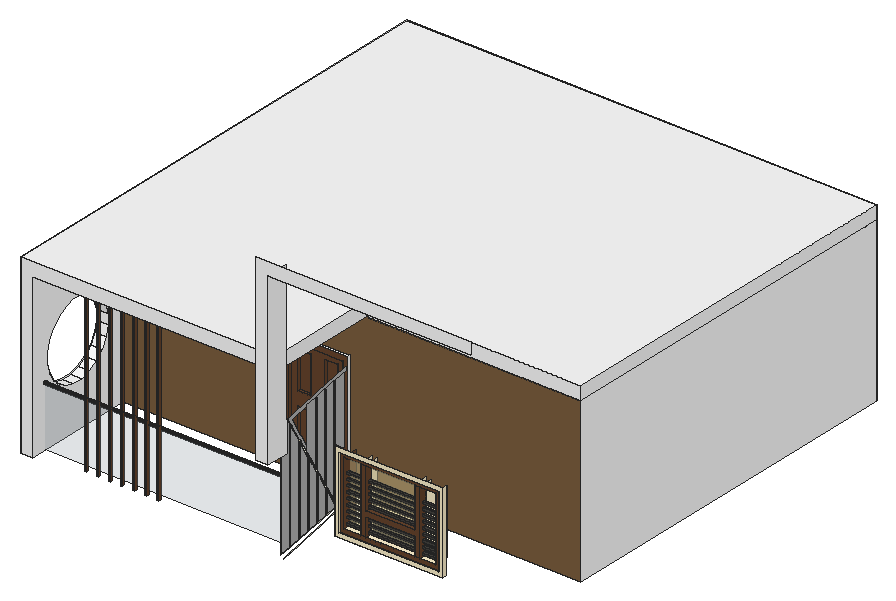
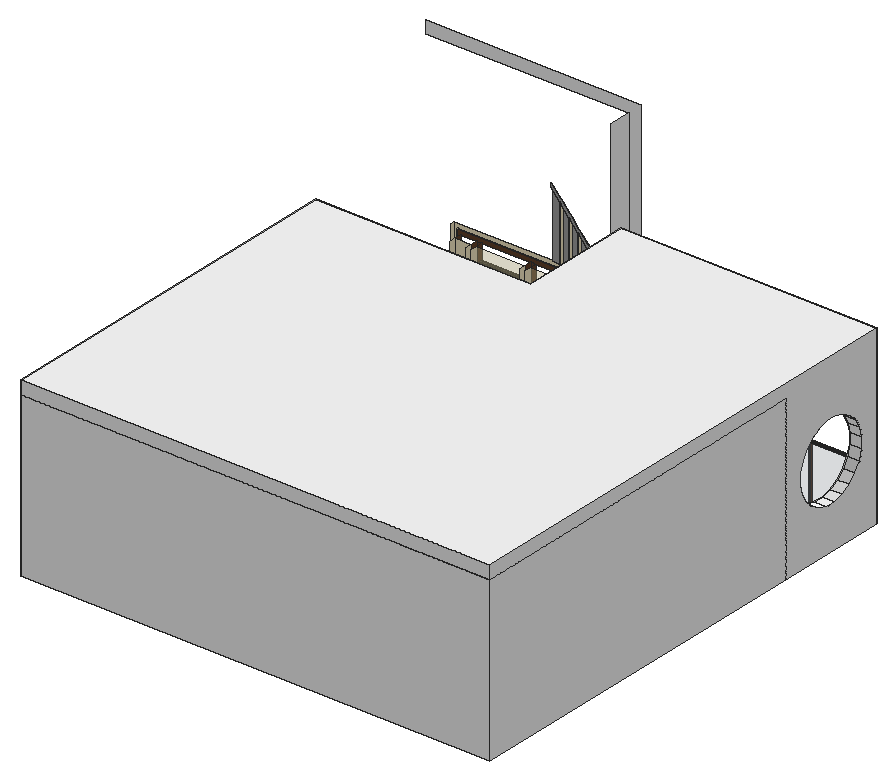
# SketchUp Ruby script. Lengths in inches.
U = 1.inch
M = Sketchup.active_model
def pt(a) = Geom::Point3d.new(a.map { |v| v * U })
def face(e, loops, mat)
  f = e.add_face(loops[0].map { |a| pt(a) })
  loops[1..].each { |l| e.add_face(l.map { |a| pt(a) }).erase! }
  f.material = f.back_material = mat if mat
  f
end
# faces: each face lists its corners as indices into pts; further lists are holes
def faces(e, pts, list, mat = nil) = list.each { |f| face(e, (f[0].is_a?(Array) ? f : [f]).map { |l| l.map { |i| pts[i] } }, mat) }
# xy, xz, yz: faces in a plane at the given z, y or x. An outline is a flat list of corners, or four numbers for a rectangle; further outlines are holes
def ring(l) = l.size == 4 ? [[l[0], l[1]], [l[2], l[1]], [l[2], l[3]], [l[0], l[3]]] : l.each_slice(2).to_a
def flat(e, list, mat, &to3) = list.each { |f| face(e, (f[0].is_a?(Array) ? f : [f]).map { |l| ring(l).map { |u, v| to3.(u, v) } }, mat) }
def xy(e, z, list, mat = nil) = flat(e, list, mat) { |x, y| [x, y, z] }
def xz(e, y, list, mat = nil) = flat(e, list, mat) { |x, z| [x, y, z] }
def yz(e, x, list, mat = nil) = flat(e, list, mat) { |y, z| [x, y, z] }
def lines(e, pts, list) = list.each { |a, b| e.add_line(pt(pts[a]), pt(pts[b])) }
# prism: a flat outline (further loops are holes) pulled along v
def prism(e, loops, v, mat = nil)
  f = face(e, loops, mat); d = Geom::Vector3d.new(v.map { |x| x * U })
  f.pushpull(f.normal.samedirection?(d) ? d.length : -d.length)
end
def box(e, o, s, mat = nil) = prism(e, [[o, [o[0] + s[0], o[1], o[2]], [o[0] + s[0], o[1] + s[1], o[2]], [o[0], o[1] + s[1], o[2]]]], [0, 0, s[2]], mat)
def at(x, y, z, deg = 0) = Geom::Transformation.translation(pt([x, y, z])) * Geom::Transformation.rotation(ORIGIN, Z_AXIS, deg.degrees)
def axes(o, x, y, z) = Geom::Transformation.new([*x, 0, *y, 0, *z, 0, *pt(o).to_a, 1])
def part(name) = M.definitions.add(name)
# library, detail: a bought-in or finely detailed component or shape, given as its bounding box
def library(name, o, s) = part(name).tap { |d| box(d.entities, o, s) }
def detail(e, o, s) = box(e.add_group.entities, o, s)
def put(e, d, t, mat = nil) = e.add_instance(d, t).tap { |i| i.material = mat if mat }
def group(e, t, mat = nil) = e.add_group.tap { |g| g.transformation = t; g.material = mat if mat }.entities
root = M.entities
M.materials.add("D01_Frost_White").color = [255, 242, 206]
M.materials.add("Glass_Basic_01").color = [161, 173, 186]
M.materials["Glass_Basic_01"].alpha = 0.25
M.materials.add("Glass_Mirror_01").color = [255, 239, 176]
M.materials["Glass_Mirror_01"].alpha = 0.4
M.materials.add("M00_Soft_Cloud").color = [255, 255, 255]
M.materials.add("M03_Pewter_Shine").color = [168, 168, 168]
M.materials.add("Metal_06_1K").color = [238, 236, 219]
M.materials.add("Plywood_01_1K").color = [125, 96, 64]
M.materials.add("Wood_Planks_01_1K").color = [69, 67, 63]
M.materials.add("Wood_Veneer_15_1K").color = [103, 69, 45]
xy(root,160,[[114.56,123.23,116,124.51],[123.54,123.23,124.98,124.51],[132.52,123.23,133.96,124.51],[141.51,123.23,142.94,124.51],[150.49,123.23,151.93,124.51],
  [159.47,123.23,160.91,124.51],[168.45,123.23,169.89,124.51]],"D01_Frost_White")
xy(root,188.68,[[307.01,114,307.01,116,312.52,116,312.52,117,313.02,117,313.02,114],[313.02,114,315.02,115],[315.02,114,387.02,117]],"D01_Frost_White")
xy(root,191.68,[[310.01,114,384.02,115.54]],"D01_Frost_White")
xy(root,194.68,[[313.01,115.54,313.02,126],[313.02,115.54,325.01,120.77],[329.01,115.54,365.01,120.77],[369.01,115.54,381.02,120.77],[313.02,120.77,325.01,126],
  [329.01,120.77,365.01,126],[369.01,120.77,381.02,126]],"D01_Frost_White")
xy(root,196.91,[[313.01,117.13,381.02,119.15]],"Wood_Planks_01_1K")
xy(root,198.29,[[313.01,117.13,381.02,119.15]],"Wood_Planks_01_1K")
xy(root,201.16,[[313.01,117.13,382.01,119.15]],"Wood_Planks_01_1K")
xy(root,202.53,[[313.01,117.13,382.01,119.15]],"Wood_Planks_01_1K")
xy(root,205.4,[[313.01,117.13,382.01,119.15]],"Wood_Planks_01_1K")
xy(root,206.77,[[313.01,117.13,382.01,119.15]],"Wood_Planks_01_1K")
xy(root,208.1,[[329.01,120.77,365.01,126]],"D01_Frost_White")
xy(root,208.1,[[329.01,115.54,365.01,120.77]],"Wood_Veneer_15_1K")
xy(root,209.64,[[313.01,117.13,382.01,119.15]],"Wood_Planks_01_1K")
xy(root,211.01,[[313.01,117.13,382.01,119.15]],"Wood_Planks_01_1K")
xy(root,212.1,[[329.01,120.77,365.01,126]],"D01_Frost_White")
xy(root,212.1,[[329.01,115.54,365.01,120.77]],"Wood_Veneer_15_1K")
xy(root,213.88,[[313.01,117.13,382.01,119.15]],"Wood_Planks_01_1K")
xy(root,215.25,[[313.01,117.13,382.01,119.15]],"Wood_Planks_01_1K")
xy(root,218.12,[[313.01,117.13,382.01,119.15]],"Wood_Planks_01_1K")
xy(root,219.49,[[313.01,117.13,382.01,119.15]],"Wood_Planks_01_1K")
xy(root,222.36,[[313.01,117.13,382.01,119.15]],"Wood_Planks_01_1K")
xy(root,223.73,[[313.01,117.13,382.01,119.15]],"Wood_Planks_01_1K")
xy(root,226.6,[[313.01,117.13,382.01,119.15]],"Wood_Planks_01_1K")
xy(root,227.97,[[313.01,117.13,382.01,119.15]],"Wood_Planks_01_1K")
xy(root,229.42,[[261.02,99,261.02,117,266.02,117,266.02,116,270.02,116,270.02,99]],"D01_Frost_White")
xy(root,230.84,[[313.01,117.13,382.01,119.15]],"Wood_Planks_01_1K")
xy(root,232.21,[[313.01,117.13,382.01,119.15]],"Wood_Planks_01_1K")
xy(root,280,[[114.56,123.23,116,124.51],[123.54,123.23,124.98,124.51],[132.52,123.23,133.96,124.51],[141.51,123.23,142.94,124.51],[150.49,123.23,151.93,124.51],
  [159.47,123.23,160.91,124.51],[168.45,123.23,169.89,124.51]],"D01_Frost_White")
xz(root,99,[[261.02,229.42,270.02,229.42,270.02,355,420.02,355,420.02,364,261.02,364]],"M00_Soft_Cloud")
xz(root,114,[[[307.01,188.68,387.02,248.68],[310.01,191.68,384.02,245.68]]],"D01_Frost_White")
xz(root,115,[[307.01,210.4375,307.01,248.68,313.02,248.68,313.02,298.84,306.31,291.09,306.31,211.3],[305.81,211.91,305.81,290.52,299.59,283.35,299.59,219.51],[299.09,220.125,299.09,282.77,292.88,275.6,292.88,227.72],[292.38,228.33,292.38,275.02,286.17,267.85,286.17,235.93]],"M03_Pewter_Shine")
xz(root,115.54,[[[310.01,191.68,384.02,245.68],[313.01,194.68,381.02,242.68]],[325.01,194.68,329.01,194.68,329.01,208.1,365.01,208.1,365.01,194.68,369.01,194.68,369.01,242.68,365.01,242.68,365.01,212.1,329.01,212.1,329.01,242.68,325.01,242.68]],"Wood_Veneer_15_1K")
xz(root,116,[[266.02,160.9375,272.24,167.99,272.24,249.17,270.02,251.83,270.02,229.42,266.02,229.42],[272.74,168.55,278.95,175.6,278.95,241.12,272.74,248.57],[279.45,176.17,285.67,183.22,285.67,233.06,279.45,240.52],[286.17,183.79,292.38,190.84,292.38,225,286.17,232.46],[292.88,191.4,299.09,198.46,299.09,216.94,292.88,224.4],
  [299.59,199.02,305.81,206.07,305.81,208.88,299.59,216.34]],"M03_Pewter_Shine")
xz(root,117,[[272.24,167.99,272.74,168.55,272.74,248.57,272.24,249.17],[278.95,175.6,279.45,176.17,279.45,240.52,278.95,241.12],[285.67,183.22,286.17,183.79,286.17,232.46,285.67,233.06],[292.38,190.84,292.88,191.4,292.88,224.4,292.38,225],[299.09,198.46,299.59,199.02,299.59,216.34,299.09,216.94],
  [305.81,206.07,306.31,206.64,306.31,208.28,305.81,208.88],[306.31,206.64,307.01,207.4375,306.31,208.28],[306.31,211.3,306.31,291.09,305.81,290.52,305.81,211.91],[299.59,219.51,299.59,283.35,299.09,282.77,299.09,220.125],[292.88,227.72,292.88,275.6,292.38,275.02,292.38,228.33]],"D01_Frost_White")
xz(root,117,[[307.01,207.4375,307.01,210.4375,306.31,211.3,305.81,211.91,299.59,219.51,299.09,220.125,292.88,227.72,292.38,228.33,286.17,235.93,285.67,236.55,279.45,244.15,278.95,244.76,272.74,252.36,278.95,259.53,279.45,260.1,285.67,267.27,286.17,267.85,292.38,275.02,292.88,275.6,299.09,282.77,299.59,283.35,305.81,290.52,306.31,291.09,313.02,298.84,313.02,301.84,306.31,294.03,305.81,293.45,299.59,286.22,299.09,285.64,292.88,278.41,292.38,277.83,286.17,270.61,285.67,270.02,279.45,262.8,278.95,262.22,272.74,254.99,272.24,254.41,270.02,251.83,272.24,249.17,272.74,248.57,278.95,241.12,279.45,240.52,285.67,233.06,286.17,232.46,292.38,225,292.88,224.4,299.09,216.94,299.59,216.34,305.81,208.88,306.31,208.28]],"M03_Pewter_Shine")
xz(root,117.13,[[313.01,196.91,381.02,198.29],[313.01,201.16,382.01,202.53],[313.01,205.4,382.01,206.77],[313.01,209.64,382.01,211.01],[313.01,213.88,382.01,215.25],
  [313.01,218.12,382.01,219.49],[313.01,222.36,382.01,223.73],[313.01,226.6,382.01,227.97],[313.01,230.84,382.01,232.21]],"Wood_Planks_01_1K")
xz(root,119.15,[[313.01,196.91,381.02,198.29],[313.01,201.16,382.01,202.53],[313.01,205.4,382.01,206.77],[313.01,209.64,382.01,211.01],[313.01,213.88,382.01,215.25],
  [313.01,218.12,382.01,219.49],[313.01,222.36,382.01,223.73],[313.01,226.6,382.01,227.97],[313.01,230.84,382.01,232.21]],"Wood_Planks_01_1K")
xz(root,120.77,[[369.01,194.68,381.02,242.68]],"D01_Frost_White")
xz(root,120.77,[[313.02,194.68,325.01,242.68],[329.01,194.68,365.01,208.1],[329.01,212.1,365.01,242.68]],"Glass_Mirror_01")
xz(root,123.23,[[114.56,160,116,280],[123.54,160,124.98,280],[132.52,160,133.96,280],[141.51,160,142.94,280],[150.49,160,151.93,280],
  [159.47,160,160.91,280],[168.45,160,169.89,280]],"Wood_Veneer_15_1K")
xz(root,124.51,[[114.56,160,116,280],[123.54,160,124.98,280],[132.52,160,133.96,280],[141.51,160,142.94,280],[150.49,160,151.93,280],
  [159.47,160,160.91,280],[168.45,160,169.89,280]],"D01_Frost_White")
yz(root,114.56,[[123.23,160,124.51,280]],"Wood_Veneer_15_1K")
yz(root,116,[[123.23,160,124.51,280]],"Wood_Veneer_15_1K")
yz(root,123.54,[[123.23,160,124.51,280]],"Wood_Veneer_15_1K")
yz(root,124.98,[[123.23,160,124.51,280]],"Wood_Veneer_15_1K")
yz(root,132.52,[[123.23,160,124.51,280]],"Wood_Veneer_15_1K")
yz(root,133.96,[[123.23,160,124.51,280]],"Wood_Veneer_15_1K")
yz(root,141.51,[[123.23,160,124.51,280]],"Wood_Veneer_15_1K")
yz(root,142.94,[[123.23,160,124.51,280]],"Wood_Veneer_15_1K")
yz(root,150.49,[[123.23,160,124.51,280]],"Wood_Veneer_15_1K")
yz(root,151.93,[[123.23,160,124.51,280]],"Wood_Veneer_15_1K")
yz(root,159.47,[[123.23,160,124.51,280]],"Wood_Veneer_15_1K")
yz(root,160.91,[[123.23,160,124.51,280]],"Wood_Veneer_15_1K")
yz(root,168.45,[[123.23,160,124.51,280]],"Wood_Veneer_15_1K")
yz(root,169.89,[[123.23,160,124.51,280]],"Wood_Veneer_15_1K")
yz(root,266.02,[[116,160.9375,117,229.42]],"D01_Frost_White")
yz(root,270.02,[[99,229.42,116,229.42,116,251.83,115,251.83,115,355,99,355]],"M00_Soft_Cloud")
yz(root,272.24,[[116,167.99,117,229.42],[116,229.42,117,249.17]],"D01_Frost_White")
yz(root,272.74,[[116,168.55,117,229.42],[116,229.42,117,248.57]],"D01_Frost_White")
yz(root,278.95,[[116,175.6,117,229.42],[116,229.42,117,241.12]],"D01_Frost_White")
yz(root,279.45,[[116,176.17,117,229.42],[116,229.42,117,240.52]],"D01_Frost_White")
yz(root,285.67,[[116,183.22,117,229.42],[116,229.42,117,233.06]],"D01_Frost_White")
yz(root,286.17,[[116,183.79,117,229.42],[116,229.42,117,232.46]],"D01_Frost_White")
yz(root,292.38,[[116,190.84,117,225],[115,228.33,117,229.42],[115,229.42,117,275.02]],"D01_Frost_White")
yz(root,292.88,[[116,191.4,117,224.4],[115,227.72,117,229.42],[115,229.42,117,275.6]],"D01_Frost_White")
yz(root,299.09,[[116,198.46,117,216.94],[115,220.125,117,229.42],[115,229.42,117,282.77]],"D01_Frost_White")
yz(root,299.59,[[116,199.02,117,216.34],[115,219.51,117,229.42],[115,229.42,117,283.35]],"D01_Frost_White")
yz(root,305.81,[[116,206.07,117,208.88],[115,211.91,117,229.42],[115,229.42,117,290.52]],"D01_Frost_White")
yz(root,306.31,[[115,211.3,117,229.42],[115,229.42,117,291.09]],"D01_Frost_White")
yz(root,307.01,[[114,188.68,114,248.68,115,248.68,115,210.4375,117,210.4375,117,204.4375,116,204.4375,116,188.68]],"D01_Frost_White")
yz(root,310.01,[[114,191.68,115.54,245.68]],"D01_Frost_White")
yz(root,313.01,[[[115.54,194.68,126,242.68],[117.13,235.08,119.15,236.46],[117.13,230.84,119.15,232.21],[117.13,226.6,119.15,227.97],[117.13,218.12,119.15,219.49],[117.13,213.88,119.15,215.25],[117.13,209.64,119.15,211.01],[117.13,201.16,119.15,202.53],[117.13,196.91,119.15,198.29],[117.13,239.33,119.15,240.7],[117.13,222.36,119.15,223.73],[117.13,205.4,119.15,206.77]]],"Wood_Veneer_15_1K")
yz(root,325.01,[[120.77,194.68,126,242.68]],"D01_Frost_White")
yz(root,325.01,[[115.54,194.68,120.77,242.68]],"Wood_Veneer_15_1K")
yz(root,329.01,[[120.77,194.68,126,208.1],[120.77,212.1,126,242.68]],"D01_Frost_White")
yz(root,329.01,[[115.54,194.68,120.77,208.1],[115.54,212.1,120.77,242.68]],"Wood_Veneer_15_1K")
yz(root,365.01,[[115.54,194.68,120.77,208.1],[120.77,194.68,126,208.1],[120.77,212.1,126,242.68]],"D01_Frost_White")
yz(root,365.01,[[115.54,212.1,120.77,242.68]],"Wood_Veneer_15_1K")
yz(root,369.01,[[120.77,194.68,126,242.68]],"D01_Frost_White")
yz(root,369.01,[[115.54,194.68,120.77,242.68]],"Wood_Veneer_15_1K")
yz(root,381.02,[[120.77,194.68,126,242.68]],"D01_Frost_White")
yz(root,381.02,[[[115.54,194.68,120.77,242.68],[117.13,196.91,119.15,198.29]]],"Wood_Veneer_15_1K")
yz(root,382.01,[[117.13,201.16,119.15,202.53],[117.13,205.4,119.15,206.77],[117.13,209.64,119.15,211.01],[117.13,213.88,119.15,215.25],[117.13,218.12,119.15,219.49],
  [117.13,222.36,119.15,223.73],[117.13,226.6,119.15,227.97],[117.13,230.84,119.15,232.21]],"Wood_Planks_01_1K")
yz(root,384.02,[[114,191.68,115.54,245.68]],"D01_Frost_White")
yz(root,387.02,[[114,188.68,117,248.68]],"D01_Frost_White")
p = [[267.98,116,159.1],[272.24,116,164.05],[272.24,117,164.05],[267.98,117,159.1],[81.02,128.05,204.61],[81.02,128.05,160],
  [261.02,128.12,160],[261.02,128.12,204.61],[272.24,116,167.99],[266.02,116,160.9375],[266.02,117,160.9375],[272.24,117,167.99],
  [272.74,116,164.625],[278.95,116,171.84],[278.95,117,171.84],[272.74,117,164.625],[278.95,116,175.6],[272.74,116,168.55],
  [272.74,117,168.55],[278.95,117,175.6],[279.45,116,172.42],[285.67,116,179.64],[285.67,117,179.64],[279.45,117,172.42],
  [285.67,116,183.22],[279.45,116,176.17],[279.45,117,176.17],[285.67,117,183.22],[286.17,116,180.22],[292.38,116,187.44],
  [292.38,117,187.44],[286.17,117,180.22],[292.38,116,190.84],[286.17,116,183.79],[286.17,117,183.79],[292.38,117,190.84],
  [292.88,116,188.02],[299.09,116,195.24],[299.09,117,195.24],[292.88,117,188.02],[299.09,116,198.46],[292.88,116,191.4],
  [292.88,117,191.4],[299.09,117,198.46],[299.59,116,195.82],[305.81,116,203.04],[305.81,117,203.04],[299.59,117,195.82],
  [305.81,116,206.07],[299.59,116,199.02],[299.59,117,199.02],[305.81,117,206.07],[306.31,116,203.62],[307.01,116,204.4375],
  [307.01,117,204.4375],[306.31,117,203.62],[299.59,116,216.34],[305.81,116,208.88],[305.81,117,208.88],[299.59,117,216.34],
  [307.01,115,210.4375],[306.31,115,211.3],[306.31,117,211.3],[307.01,117,210.4375],[305.81,115,211.91],[299.59,115,219.51],
  [299.59,117,219.51],[305.81,117,211.91],[292.88,116,224.4],[299.09,116,216.94],[299.09,117,216.94],[292.88,117,224.4],
  [299.09,115,220.125],[292.88,115,227.72],[292.88,117,227.72],[299.09,117,220.125],[286.17,116,232.46],[292.38,116,225],
  [292.38,117,225],[286.17,117,232.46],[292.38,115,228.33],[286.17,115,235.93],[286.17,117,235.93],[292.38,117,228.33],
  [279.45,116,240.52],[285.67,116,233.06],[285.67,117,233.06],[279.45,117,240.52],[312.52,117,229.42],[312.52,117,188.68],
  [313.02,117,194.68],[313.02,117,188.68]]
faces(root,p,[[0,1,2,3],[8,9,10,11],[12,13,14,15],[16,17,18,19],[20,21,22,23],[24,25,26,27],[28,29,30,31],[32,33,34,35],
  [36,37,38,39],[40,41,42,43],[44,45,46,47],[48,49,50,51],[52,53,54,55],[56,57,58,59],[60,61,62,63],[64,65,66,67],
  [68,69,70,71],[72,73,74,75],[76,77,78,79],[80,81,82,83],[84,85,86,87]],"Metal_06_1K")
faces(root,p,[[4,5,6,7]],"Glass_Basic_01")
lines(root,p,[[88,89],[90,91]])
g1 = group(root,at(72.02,201,160),"M00_Soft_Cloud")
xy(g1,0,[[9,9,341.95,264.44]])
xy(g1,6,[[129,-2,177,0]])
xy(g1,10,[[133,-2,173,0]],"Wood_Veneer_15_1K")
xy(g1,15,[[138,0,148,2],[158,0,168,2]],"Wood_Veneer_15_1K")
xy(g1,43,[[138,0,148,2],[158,0,168,2]],"Wood_Veneer_15_1K")
xy(g1,53,[[138,0,148,2],[158,0,168,2]],"Wood_Veneer_15_1K")
xy(g1,81,[[138,0,148,2],[158,0,168,2]],"Wood_Veneer_15_1K")
xy(g1,86,[[133,-2,173,0]],"Wood_Veneer_15_1K")
xy(g1,90,[[129,-2,177,0]])
xy(g1,120,[[[0,0,348,273.44],[9,9,341.95,264.44]]])
xz(g1,-2,[[[129,6,177,90],[133,10,173,86]]],"Wood_Veneer_15_1K")
xz(g1,0,[[[0,0,348,120],[129,6,177,90]]],"Plywood_01_1K")
xz(g1,0,[[[133,10,173,86],[158,53,168,81],[138,15,148,43],[138,53,148,81],[158,15,168,43]]],"Wood_Veneer_15_1K")
xz(g1,2,[[138,15,148,43],[158,15,168,43],[138,53,148,81],[158,53,168,81]],"Wood_Veneer_15_1K")
xz(g1,9,[[9,0,341.95,120]])
xz(g1,264.44,[[9,0,341.95,120]])
xz(g1,273.44,[[0,0,348,120]])
yz(g1,0,[[0,0,273.44,120]])
yz(g1,9,[[9,0,264.44,120]])
yz(g1,129,[[-2,6,0,90]])
yz(g1,133,[[-2,10,0,86]],"Wood_Veneer_15_1K")
yz(g1,138,[[0,15,2,43],[0,53,2,81]],"Wood_Veneer_15_1K")
yz(g1,148,[[0,15,2,43],[0,53,2,81]],"Wood_Veneer_15_1K")
yz(g1,158,[[0,15,2,43],[0,53,2,81]],"Wood_Veneer_15_1K")
yz(g1,168,[[0,15,2,43],[0,53,2,81]],"Wood_Veneer_15_1K")
yz(g1,173,[[-2,10,0,86]],"Wood_Veneer_15_1K")
yz(g1,177,[[-2,6,0,90]])
yz(g1,341.95,[[9,0,264.44,120]])
yz(g1,348,[[0,0,273.44,120]])
g2 = group(root,at(81.02,210,280),"M00_Soft_Cloud")
xy(g2,-120,[[-9,-93,0,-9]])
xy(g2,0,[[0,-93,0,-9,-9,-9,-9,264.44,339,264.44,339,-9,180,-9,180,-93]])
xy(g2,10,[[-9,-93,180,-93,180,-9,339,-9,339,264.44,-9,264.44]])
xz(g2,-93,[[-9,-120,0,-120,0,0,180,0,180,10,-9,10]])
xz(g2,-9,[[-9,-120,0,0],[180,0,339,10]])
xz(g2,264.44,[[-9,0,339,10]])
yz(g2,-9,[[[-93,-120,-93,10,264.44,10,264.44,0,-9,0,-9,-120],[-54.27,-88.27,-46.77,-88.14,-39.5625,-86.08,-33.13,-82.22,-27.92,-76.83,-24.29,-70.27,-22.47,-62.99,-22.6,-55.5,-24.66,-48.29,-28.52,-41.86,-33.91,-36.65,-40.47,-33.01,-47.75,-31.19,-55.24,-31.32,-62.45,-33.39,-68.88,-37.25,-74.09,-42.64,-77.73,-49.2,-79.55,-56.47,-79.42,-63.97,-77.36,-71.18,-73.5,-77.61,-68.1,-82.82,-61.55,-86.45]]])
yz(g2,0,[[[-93,-120,-9,0],[-54.27,-88.27,-61.55,-86.45,-68.1,-82.82,-73.5,-77.61,-77.36,-71.18,-79.42,-63.97,-79.55,-56.47,-77.73,-49.2,-74.09,-42.64,-68.88,-37.25,-62.45,-33.39,-55.24,-31.32,-47.75,-31.19,-40.47,-33.01,-33.91,-36.65,-28.52,-41.86,-24.66,-48.29,-22.6,-55.5,-22.47,-62.99,-24.29,-70.27,-27.92,-76.83,-33.13,-82.22,-39.5625,-86.08,-46.77,-88.14],[-82.39,-75.51,-82.62,-75.48,-82.83,-75.39,-83.01,-75.25,-83.15,-75.0625,-83.24,-74.85,-83.27,-74.62,-83.24,-74.39,-83.15,-74.18,-83.01,-74,-82.83,-73.86,-82.62,-73.77,-82.39,-73.74,-82.16,-73.77,-81.95,-73.86,-81.76,-74,-81.62,-74.18,-81.53,-74.39,-81.5,-74.62,-81.53,-74.85,-81.62,-75.0625,-81.76,-75.25,-81.95,-75.39,-82.16,-75.48]]])
yz(g2,180,[[-82.39,-75.51,-82.16,-75.48,-81.95,-75.39,-81.76,-75.25,-81.62,-75.0625,-81.53,-74.85,-81.5,-74.62,-81.53,-74.39,-81.62,-74.18,-81.76,-74,-81.95,-73.86,-82.16,-73.77,-82.39,-73.74,-82.62,-73.77,-82.83,-73.86,-83.01,-74,-83.15,-74.18,-83.24,-74.39,-83.27,-74.62,-83.24,-74.85,-83.15,-75.0625,-83.01,-75.25,-82.83,-75.39,-82.62,-75.48],[-93,0,-9,10]])
yz(g2,339,[[-9,0,264.44,10]])
p = [[0,-61.55,-86.45],[0,-54.27,-88.27],[-9,-54.27,-88.27],[-9,-61.55,-86.45],[0,-46.77,-88.14],[-9,-46.77,-88.14],
  [0,-39.5625,-86.08],[-9,-39.5625,-86.08],[0,-68.1,-82.82],[-9,-68.1,-82.82],[0,-33.13,-82.22],[-9,-33.13,-82.22],
  [0,-73.5,-77.61],[-9,-73.5,-77.61],[0,-27.92,-76.83],[-9,-27.92,-76.83],[0,-77.36,-71.18],[-9,-77.36,-71.18],
  [0,-24.29,-70.27],[-9,-24.29,-70.27],[0,-82.83,-75.39],[0,-82.62,-75.48],[180,-82.62,-75.48],[180,-82.83,-75.39],
  [0,-82.39,-75.51],[180,-82.39,-75.51],[0,-82.16,-75.48],[180,-82.16,-75.48],[0,-81.95,-75.39],[180,-81.95,-75.39],
  [0,-83.01,-75.25],[180,-83.01,-75.25],[0,-81.76,-75.25],[180,-81.76,-75.25],[0,-83.15,-75.0625],[180,-83.15,-75.0625],
  [0,-81.62,-75.0625],[180,-81.62,-75.0625],[0,-83.24,-74.85],[180,-83.24,-74.85],[0,-81.53,-74.85],[180,-81.53,-74.85],
  [0,-83.27,-74.62],[180,-83.27,-74.62],[0,-81.5,-74.62],[180,-81.5,-74.62],[0,-83.24,-74.39],[180,-83.24,-74.39],
  [0,-81.53,-74.39],[180,-81.53,-74.39],[0,-83.15,-74.18],[180,-83.15,-74.18],[0,-81.62,-74.18],[180,-81.62,-74.18],
  [0,-83.01,-74],[180,-83.01,-74],[0,-81.76,-74],[180,-81.76,-74],[0,-82.83,-73.86],[180,-82.83,-73.86],
  [0,-81.95,-73.86],[180,-81.95,-73.86],[0,-82.62,-73.77],[180,-82.62,-73.77],[0,-82.16,-73.77],[180,-82.16,-73.77],
  [0,-82.39,-73.74],[180,-82.39,-73.74],[0,-79.42,-63.97],[-9,-79.42,-63.97],[0,-22.47,-62.99],[-9,-22.47,-62.99],
  [0,-79.55,-56.47],[-9,-79.55,-56.47],[0,-22.6,-55.5],[-9,-22.6,-55.5],[0,-77.73,-49.2],[-9,-77.73,-49.2],
  [0,-24.66,-48.29],[-9,-24.66,-48.29],[0,-74.09,-42.64],[-9,-74.09,-42.64],[0,-28.52,-41.86],[-9,-28.52,-41.86],
  [0,-68.88,-37.25],[-9,-68.88,-37.25],[0,-33.91,-36.65],[-9,-33.91,-36.65],[0,-62.45,-33.39],[-9,-62.45,-33.39],
  [0,-40.47,-33.01],[-9,-40.47,-33.01],[0,-55.24,-31.32],[-9,-55.24,-31.32],[0,-47.75,-31.19],[-9,-47.75,-31.19]]
faces(g2,p,[[0,1,2,3],[1,4,5,2],[4,6,7,5],[8,0,3,9],[6,10,11,7],[12,8,9,13],[10,14,15,11],[16,12,13,17],
  [14,18,19,15],[20,21,22,23],[21,24,25,22],[24,26,27,25],[26,28,29,27],[30,20,23,31],[28,32,33,29],[34,30,31,35],
  [32,36,37,33],[38,34,35,39],[36,40,41,37],[42,38,39,43],[40,44,45,41],[46,42,43,47],[44,48,49,45],[50,46,47,51],
  [48,52,53,49],[54,50,51,55],[52,56,57,53],[58,54,55,59],[56,60,61,57],[62,58,59,63],[60,64,65,61],[66,62,63,67],
  [64,66,67,65],[68,16,17,69],[18,70,71,19],[72,68,69,73],[70,74,75,71],[76,72,73,77],[74,78,79,75],[80,76,77,81],
  [78,82,83,79],[84,80,81,85],[82,86,87,83],[88,84,85,89],[86,90,91,87],[92,88,89,93],[90,94,95,91],[94,92,93,95]])
